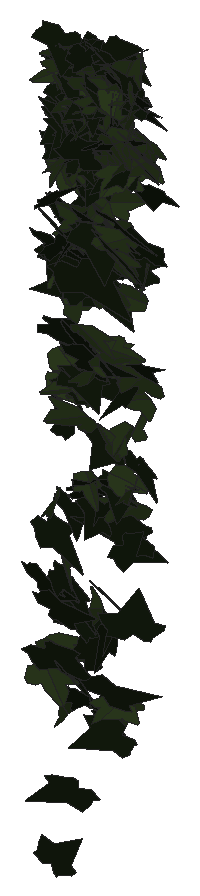
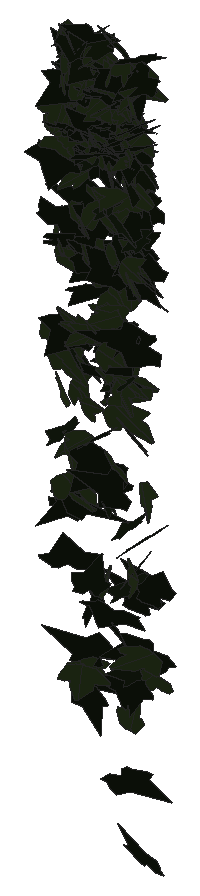
# SketchUp Ruby script. Lengths in millimetres.
U = 1.mm
M = Sketchup.active_model
def pt(a) = Geom::Point3d.new(a.map { |v| v * U })
def face(e, loops, mat)
  f = e.add_face(loops[0].map { |a| pt(a) })
  loops[1..].each { |l| e.add_face(l.map { |a| pt(a) }).erase! }
  f.material = f.back_material = mat if mat
  f
end
# faces: each face lists its corners as indices into pts; further lists are holes
def faces(e, pts, list, mat = nil) = list.each { |f| face(e, (f[0].is_a?(Array) ? f : [f]).map { |l| l.map { |i| pts[i] } }, mat) }
# xy, xz, yz: faces in a plane at the given z, y or x. An outline is a flat list of corners, or four numbers for a rectangle; further outlines are holes
def ring(l) = l.size == 4 ? [[l[0], l[1]], [l[2], l[1]], [l[2], l[3]], [l[0], l[3]]] : l.each_slice(2).to_a
def flat(e, list, mat, &to3) = list.each { |f| face(e, (f[0].is_a?(Array) ? f : [f]).map { |l| ring(l).map { |u, v| to3.(u, v) } }, mat) }
def xy(e, z, list, mat = nil) = flat(e, list, mat) { |x, y| [x, y, z] }
def xz(e, y, list, mat = nil) = flat(e, list, mat) { |x, z| [x, y, z] }
def yz(e, x, list, mat = nil) = flat(e, list, mat) { |y, z| [x, y, z] }
def lines(e, pts, list) = list.each { |a, b| e.add_line(pt(pts[a]), pt(pts[b])) }
# prism: a flat outline (further loops are holes) pulled along v
def prism(e, loops, v, mat = nil)
  f = face(e, loops, mat); d = Geom::Vector3d.new(v.map { |x| x * U })
  f.pushpull(f.normal.samedirection?(d) ? d.length : -d.length)
end
def box(e, o, s, mat = nil) = prism(e, [[o, [o[0] + s[0], o[1], o[2]], [o[0] + s[0], o[1] + s[1], o[2]], [o[0], o[1] + s[1], o[2]]]], [0, 0, s[2]], mat)
def at(x, y, z, deg = 0) = Geom::Transformation.translation(pt([x, y, z])) * Geom::Transformation.rotation(ORIGIN, Z_AXIS, deg.degrees)
def axes(o, x, y, z) = Geom::Transformation.new([*x, 0, *y, 0, *z, 0, *pt(o).to_a, 1])
def part(name) = M.definitions.add(name)
# library, detail: a bought-in or finely detailed component or shape, given as its bounding box
def library(name, o, s) = part(name).tap { |d| box(d.entities, o, s) }
def detail(e, o, s) = box(e.add_group.entities, o, s)
def put(e, d, t, mat = nil) = e.add_instance(d, t).tap { |i| i.material = mat if mat }
def group(e, t, mat = nil) = e.add_group.tap { |g| g.transformation = t; g.material = mat if mat }.entities
root = M.entities
M.materials.add("efeu1").color = [18, 25, 13]
M.materials.add("efeu2").color = [43, 57, 29]
c1 = part("ivyleaf_10")
p = [[0,12.8,-0.8],[-1.5,51.3,-10.9],[-4.9,51,-11.6],[-13.6,26.5,-7.3],[-13.2,15.9,-4.6],[-21.1,19.3,-7.2],
  [-29.5,16.3,-8.3],[-29.2,8.3,-6.2],[-19.7,-9.8,0.5],[-7.6,-13,4],[1,-12.2,5.8],[-0.4,51.1,-11.1],
  [-1.5,51.1,-10.9],[1,-12.4,5.9],[16.9,-12.4,3.5],[35.1,9.1,-5.1],[35,12.9,-6.1],[20.5,16.4,-4.9],
  [15.8,15,-3.8],[15.3,27.6,-7.1],[12.8,31.3,-7.8]]
faces(c1.entities,p,[[0,1,2,3,4,5,6,7,8,9,10],[11,12,0,13,14,15,16,17,18,19,20]],"efeu2")
c2 = part("ivyleaf_9")
p = [[39.1,54.8,31.7],[34.5,51.8,30.2],[-5.3,25.2,17.3],[-17.9,28.3,20.9],[-21.6,21.7,17],[-20.2,4.3,5.3],
  [-22.9,-0.3,2.5],[-17.1,-4,-0.6],[-2,-2.1,-1.2],[-0.7,-15.4,-10.1],[16.6,-22.3,-16.7],[21.1,-15.1,-12.5],
  [32.7,-10.7,-11],[46.1,-1.8,-6.6],[30.8,11.2,3.8]]
faces(c2.entities,p,[[0,1,2,3,4,5,6,7,8,9,10,11,12,13,14]],"efeu1")
put(root,c1,axes([2672.7,935.9,813.4],[0.15942,-0.86743,-0.26606],[-0.00895,0.26677,-0.87123],[1.72677,0.08147,0.02005]))
put(root,c2,axes([2720.5,938.2,1232.8],[-0.34672,-0.3779,-0.92751],[1.32636,0.62923,-0.39325],[1.36897,-0.70536,0.1461]))
put(root,c2,axes([2660.8,944.4,613.2],[0.17561,-0.06532,0.79458],[1.07748,-0.55783,-0.1116],[1.06836,0.57333,-0.01806]))
put(root,c2,axes([2787.7,950.3,434.8],[-1.28493,-0.29658,0.36083],[-0.63314,-0.13984,-0.7374],[0.62397,-0.75264,-0.00518]))
put(root,c1,axes([2677.2,946.4,1400.3],[0.03085,-0.75073,0.26481],[0.10097,-0.26326,-0.74957],[1.5117,0.0329,0.04466]))
put(root,c1,axes([2790.3,937.7,1478.8],[-1.40891,0.26566,-0.16374],[0.28464,-0.06793,-0.7864],[-0.52128,-0.75513,0.01314]))
put(root,c1,axes([2797,954.6,969.3],[-0.08285,-0.6242,0.55645],[0.28955,-0.55382,-0.60934],[1.56493,0.06942,0.1422]))
put(root,c1,axes([2822.4,927,1490],[0.29713,-0.25999,0.8628],[-0.7831,0.75847,0.303],[-1.52579,-0.43991,0.01251]))
put(root,c2,axes([2666.2,956.2,1276.6],[1.22665,-0.55319,-0.25391],[0.36613,-0.16572,0.84937],[-1.09906,-0.67262,-0.00044]))
put(root,c2,axes([2673.5,937.4,685.2],[0.65802,-0.47064,-0.52274],[-0.59753,0.41797,-0.58398],[1.19795,0.467,-0.00415]))
put(root,c2,axes([2657,928.9,1336.1],[0.09252,0.6858,-0.38367],[-0.11219,0.3865,0.6834],[1.49137,-0.01347,0.07521]))
put(root,c2,axes([2628.6,954.2,644.9],[0.27741,-0.22383,0.84752],[0.86326,-0.71593,-0.26709],[1.42759,0.47642,-0.00318]))
put(root,c1,axes([2702.9,956.9,1013.9],[-0.17582,-0.23371,0.79373],[-0.68279,-0.70837,-0.25033],[1.41902,-0.3698,-0.02211]))
put(root,c2,axes([2714.2,947.5,1067.5],[0.49529,-0.17699,0.81736],[1.30688,-0.44341,-0.31464],[0.90854,0.7343,0.00701]))
put(root,c1,axes([2725,942.1,1487.2],[0.18277,-0.80694,-0.22992],[-0.07025,0.22713,-0.81258],[1.59534,0.10245,-0.00944]))
put(root,c1,axes([2733.9,946.2,1050.5],[-0.37143,-0.74584,0.00108],[0.00403,-0.00167,-0.77095],[1.41948,-0.19516,0.00247]))
put(root,c2,axes([2716,947.6,1045.3],[-0.36467,-0.63332,-0.39148],[0.2294,0.37252,-0.66164],[1.39834,-0.22628,0.00645]))
put(root,c2,axes([2740.4,936.6,1617.8],[-0.89527,0.69738,0.26632],[-0.25461,0.23093,-0.84102],[-1.39773,-0.48875,-0.01738]))
put(root,c2,axes([2823.1,941,632.2],[-1.18983,-0.33633,0.57308],[1.1117,0.09693,0.69411],[-0.60287,0.84253,0.14891]))
put(root,c1,axes([2783.9,955.2,1533.3],[-0.17063,-0.77778,0.38312],[0.07826,-0.38854,-0.77916],[1.64824,-0.06207,0.07666]))
put(root,c1,axes([2826.6,929.7,1566.8],[0.06729,-0.15347,-0.87719],[-0.05514,0.87721,-0.15465],[1.69392,0.03465,0.02981]))
put(root,c2,axes([2787.1,958.1,1561.1],[-0.0691,-0.36872,0.77727],[0.87035,-0.66722,-0.29515],[1.38682,0.40036,0.22396]))
put(root,c2,axes([2709.5,947.5,1195.5],[-1.3001,0.31373,0.19461],[-0.34843,0.06757,-0.75157],[-0.61016,-0.70707,0.01452]))
put(root,c2,axes([2714.3,957.1,1463.5],[-1.48201,-0.3229,0.02286],[-0.03599,-0.01406,-0.84297],[0.61503,-0.7789,0.00574]))
put(root,c2,axes([2722.7,937.8,1429.1],[-0.27769,-0.00995,0.93928],[1.75685,0.17443,0.14524],[-0.33092,0.93441,-0.01711]))
put(root,c1,axes([2680.4,955.1,1564.4],[0.7392,0.38225,-0.66317],[-1.11093,-0.33316,-0.5339],[-0.9424,0.69257,0.10919]))
put(root,c2,axes([2731.9,945,1104],[1.36557,-0.37346,-0.34054],[-0.57379,0.15835,-0.80889],[0.77202,0.77828,0.00117]))
put(root,c2,axes([2723.4,949,548],[-0.37124,0.65819,0.57866],[0.2768,-0.56029,0.68632],[1.64482,0.24284,0.01511]))
put(root,c1,axes([2731.1,947.6,1560.2],[-1.35513,-0.2036,-0.34563],[0.65126,0.05915,-0.73979],[0.39837,-0.78927,0.03372]))
put(root,c1,axes([2696,958.5,1390.3],[0.17184,-0.75813,-0.35778],[0.37363,-0.33072,0.75033],[-1.55111,-0.16365,0.14111]))
put(root,c1,axes([2742.7,958.3,1526.1],[-0.52643,-0.71406,0.32298],[-0.07957,-0.32857,-0.76224],[1.48944,-0.26993,0.07343]))
put(root,c2,axes([2758.1,961.4,1279.5],[0.70383,-0.73572,0.38608],[0.39609,-0.3271,-0.82267],[1.53089,0.42288,0.03535]))
put(root,c1,axes([2722.5,950.5,1120.3],[-1.17375,0.19329,-0.48174],[0.88305,-0.13013,-0.6462],[-0.44291,-0.77168,-0.01169]))
put(root,c1,axes([2789.3,944.2,935.7],[0.68756,-0.16034,0.68765],[-1.21035,0.26174,0.39514],[-0.58391,-0.73134,-0.00934]))
put(root,c1,axes([2803.2,956.3,1482.5],[-1.05761,-0.327,0.56889],[-0.87459,-0.33821,-0.64328],[0.89145,-0.71976,0.04381]))
put(root,c1,axes([2715.5,958.8,854.4],[1.05753,-0.26871,0.55155],[0.93717,-0.24855,-0.61718],[0.69652,0.74241,-0.007]))
put(root,c2,axes([2739.4,963.1,1287.4],[-0.41817,-0.92359,-0.06457],[0.03619,0.06185,-0.94935],[1.76169,-0.2205,0.00417]))
put(root,c2,axes([2669.8,962.9,1615.3],[-0.58633,-0.77862,-0.02139],[0.02606,0.01758,-0.83733],[1.48221,-0.30831,0.00626]))
put(root,c2,axes([2789.6,939.3,1476.3],[0.837,0.67539,0.11118],[0.10284,0.09748,-0.80591],[-1.29863,0.44302,0.00783]))
put(root,c1,axes([2643.7,953.7,491.3],[1.49892,0.11324,0.37942],[0.71659,0.04721,-0.79566],[-0.23321,0.87293,-0.00619]))
put(root,c2,axes([2736.5,962.9,1559.2],[0.36434,-0.80566,0.1529],[0.03311,-0.15299,-0.8279],[1.56036,0.19137,-0.01814]))
put(root,c1,axes([2681.9,946.8,1066.9],[0.77895,0.63903,0.34305],[0.35015,0.28954,-0.75886],[-1.33521,0.44873,0.00112]))
put(root,c2,axes([2752.8,969.4,596.9],[-0.02818,0.03185,-0.97254],[1.18631,-0.74658,-0.03394],[-1.42207,-0.62344,-0.00904]))
put(root,c2,axes([2704.8,946,1111.4],[1.33807,-0.07472,-0.51763],[-0.9718,0.08956,-0.70646],[0.21534,0.86846,0.02832]))
put(root,c2,axes([2807.2,957,1047.6],[-1.17691,0.56372,-0.46815],[0.65936,-0.31487,-0.83677],[-1.22888,-0.70882,-0.00062]))
put(root,c2,axes([2648.2,948.7,534.5],[-0.1224,-0.04493,-0.85682],[1.17092,0.59647,-0.07746],[1.13818,-0.61846,-0.01246]))
put(root,c1,axes([2782.4,960.8,1298.4],[-0.85556,-0.26961,0.57998],[-0.77328,-0.42711,-0.51347],[0.94009,-0.59669,0.10548]))
put(root,c2,axes([2783.6,958.5,1422.2],[-1.27403,0.28651,-0.3096],[0.49768,-0.17384,-0.72627],[-0.62996,-0.71677,0.05238]))
put(root,c1,axes([2782.5,958.8,1413],[1.0057,0.51896,-0.39533],[-0.58093,-0.25295,-0.74005],[-1.09733,0.60954,0.02947]))
put(root,c1,axes([2758.8,950.7,1209.2],[-1.70865,0.06043,0.2919],[-0.5547,0.01631,-0.8998],[-0.11897,-0.9439,0.00314]))
put(root,c2,axes([2759.5,961.1,1320],[0.78526,-0.46789,0.54841],[0.77524,-0.37002,-0.62216],[1.13198,0.57799,0.04565]))
put(root,c1,axes([2692.4,949.4,1557.1],[-0.80403,-0.11546,-0.7096],[1.32313,0.14407,-0.43734],[0.34858,-0.81318,0.02327]))
put(root,c1,axes([2718,953.3,1499.1],[-0.54373,-0.77837,-0.12874],[0.08638,0.12048,-0.82914],[1.49903,-0.28927,0.00108]))
put(root,c1,axes([2703.8,968.5,1305.9],[-0.72792,-0.4744,-0.72554],[-0.85098,-0.57142,0.60934],[-1.41341,0.58836,0.00679]))
put(root,c1,axes([2739.5,953.7,1448.3],[-1.22505,0.46513,-0.12795],[0.18629,-0.08298,-0.79409],[-0.89901,-0.65101,0.00981]))
put(root,c1,axes([2801.2,956.6,1612.9],[-0.82733,-0.70588,0.01715],[-0.01854,-0.01415,-0.82899],[1.3437,-0.43481,-0.00087]))
put(root,c1,axes([2760.1,946.1,1072.6],[-0.2766,-0.34891,0.74435],[0.70572,0.6468,0.37558],[-1.39634,0.39601,0.04237]))
put(root,c2,axes([2752,954.2,491.6],[0.18914,-0.0196,0.83537],[1.53631,-0.21511,-0.10108],[0.4109,0.81329,-0.00661]))
put(root,c1,axes([2783.2,942.1,1536.1],[0.44676,0.64527,-0.63514],[0.1941,0.63312,0.68091],[1.71223,-0.24014,0.08853]))
put(root,c1,axes([2827.3,956.7,1448.2],[-1.23998,0.00173,0.47916],[-0.9028,-0.11656,-0.64458],[0.1288,-0.80031,0.09491]))
put(root,c2,axes([2727.8,973.7,791.9],[-0.30813,-0.59527,0.53616],[-0.27348,-0.51655,-0.61689],[1.49999,-0.21646,-0.00234]))
put(root,c1,axes([2812.8,958.7,1203.8],[-0.16965,0.00393,-0.79023],[-1.50347,0.02042,0.08921],[0.03946,0.79498,0.00162]))
put(root,c2,axes([2689.4,966.3,299.2],[0.04421,0.06156,-0.80436],[-0.5756,-0.74534,-0.06577],[-1.42336,0.30332,0.00162]))
put(root,c2,axes([2644.2,958.3,749.8],[0.58112,-0.83208,-0.39431],[-0.20035,0.38115,-0.88583],[1.74093,0.32161,0.02968]))
put(root,c1,axes([2730.3,969.9,628.5],[-0.39409,0.37062,0.7211],[0.58023,-0.65404,0.4237],[1.42981,0.36757,0.02681]))
put(root,c2,axes([2725.3,966,1575.4],[-0.66683,-0.70614,-0.2528],[0.45866,0.15824,-0.77601],[1.35177,-0.40203,0.1386]))
put(root,c2,axes([2680.1,944,1428.1],[-0.29968,0.63778,0.51889],[-0.32559,0.49135,-0.65583],[-1.53056,-0.2294,0.03792]))
put(root,c2,axes([2804.3,968,1582.8],[-0.01937,-0.94154,0.03423],[0.01272,0.03416,0.94158],[-1.79308,0.01042,0.00631]))
put(root,c1,axes([2823.3,956.8,1068.5],[-1.62784,-0.0793,0.43208],[-0.81798,-0.04455,-0.85897],[0.17293,-0.95722,0.00418]))
put(root,c2,axes([2710.8,970.8,1521.2],[-0.10955,-0.81263,0.14807],[-0.05328,-0.14642,-0.81448],[1.57115,-0.06163,-0.0173]))
put(root,c1,axes([2772.4,964.6,474.6],[1.0681,0.4258,-0.46867],[-0.71452,-0.28056,-0.70446],[-0.97047,0.67521,0.00284]))
put(root,c1,axes([2771.3,958.1,1266.6],[-1.32442,0.12671,-0.34042],[0.61959,-0.10874,-0.70597],[-0.30663,-0.76702,0.04385]))
put(root,c2,axes([2671.3,968.8,652.7],[0.57538,-0.90792,0.12651],[0.08216,-0.11897,-0.95693],[1.74271,0.30537,0.00335]))
put(root,c2,axes([2774.8,949.6,1512.1],[0.07015,-0.37409,0.75682],[0.49263,0.72606,0.34628],[-1.52934,0.21672,0.14626]))
put(root,c2,axes([2700.2,976.1,1490.8],[-0.58174,-0.62853,0.46493],[0.15563,-0.52217,-0.65214],[1.47975,-0.19218,0.25137]))
put(root,c1,axes([2716.3,943.6,1020.7],[0.34793,0.24503,-0.78762],[0.64119,0.7142,0.30038],[1.43296,-0.37907,0.05683]))
put(root,c2,axes([2739.1,973.2,1523.8],[-1.28127,-0.40069,0.27581],[-0.30363,-0.26301,-0.77151],[0.87459,-0.67832,0.13622]))
put(root,c2,axes([2659.2,967.5,1313],[1.2524,-0.06727,-0.51152],[0.96347,-0.07573,0.66121],[-0.1894,-0.83003,-0.01888]))
put(root,c2,axes([2695.7,968.9,1286.3],[-0.64733,0.42247,-0.77528],[0.90343,-0.61303,-0.54231],[-1.41684,-0.58391,0.00842]))
put(root,c1,axes([2809.9,961.5,1530.4],[0.05668,-0.835,-0.01775],[-0.01542,0.01748,-0.83549],[1.58945,0.02995,-0.00747]))
put(root,c2,axes([2688.5,959.3,1549.6],[0.61306,-0.68183,-0.35126],[-0.14218,0.35128,-0.75038],[1.4528,0.3221,0.07479]))
put(root,c1,axes([2815.1,963.1,1617.3],[0.17058,-0.82463,0.07011],[0.44247,-0.04259,-0.79818],[1.51167,0.10552,0.22572]))
put(root,c2,axes([2802,966.3,1552.2],[-1.56301,-0.03334,-0.01598],[0.03086,-0.0054,-0.82191],[0.06324,-0.82139,0.00605]))
put(root,c1,axes([2786.7,962.7,1430.3],[-1.2637,-0.63073,0.06055],[0.09244,0.03678,0.91578],[-1.20237,0.66573,0.00677]))
put(root,c1,axes([2699.8,961.6,957.9],[-1.07253,-0.19468,0.67021],[-1.22089,-0.1948,-0.59598],[0.52317,-0.85371,-0.01684]))
put(root,c2,axes([2696.6,975.5,1015.9],[0.79633,-0.76132,-0.18772],[0.19844,-0.15686,0.86858],[-1.47908,-0.43094,0.01546]))
put(root,c1,axes([2680.7,959.4,1595.5],[-1.01355,-0.62878,-0.11069],[0.10024,0.10039,-0.82363],[1.21095,-0.53459,-0.02447]))
put(root,c2,axes([2780.8,969,1461.5],[0.7426,-0.6508,0.27175],[0.33325,-0.21145,-0.7578],[1.30023,0.42589,0.03902]))
put(root,c1,axes([2803.6,955.2,1446.8],[-0.22263,-0.72728,-0.411],[0.09085,0.40851,-0.73646],[1.58729,-0.12539,-0.01549]))
put(root,c2,axes([2678.3,948.2,1400],[0.32565,0.75323,0.1979],[0.0868,0.19258,-0.77241],[-1.47965,0.17707,-0.00175]))
put(root,c1,axes([2665.3,960.7,1474.7],[-1.40582,0.29447,-0.24979],[0.42623,-0.11254,-0.79493],[-0.59869,-0.77159,0.02061]))
put(root,c2,axes([2667.4,946.3,1258.2],[-0.12875,0.11804,-0.82061],[-0.49208,0.77927,0.13341],[1.49916,0.26592,-0.02669]))
put(root,c1,axes([2755.1,962.2,1580.5],[-1.11668,-0.60124,-0.00818],[0.00861,0.00701,-0.84008],[1.14434,-0.58675,-0.00166]))
put(root,c2,axes([2758.5,959.5,1630.4],[-0.19763,-0.39536,-0.73817],[0.73401,0.63766,-0.39578],[1.4146,-0.3861,0.10223]))
put(root,c1,axes([2676.2,963.2,1187.8],[1.00666,0.56042,-0.0564],[-0.07579,-0.03997,-0.77061],[-1.06931,0.53043,0.00153]))
put(root,c2,axes([2797.1,969.2,1557],[-1.54014,-0.03063,0.18632],[-0.35454,-0.00429,-0.80981],[0.05864,-0.8304,-0.00269]))
put(root,c2,axes([2739.3,968.7,1393.9],[-1.30451,0.07223,-0.39946],[0.76189,-0.00967,-0.68866],[-0.12807,-0.79327,-0.02798]))
put(root,c1,axes([2803.2,960.2,866.6],[-0.02823,-0.78479,-0.29344],[-0.0224,0.29365,-0.78476],[1.59445,-0.00977,-0.01622]))
put(root,c2,axes([2762.7,960.9,1459.1],[0.12892,0.75149,-0.39845],[-0.05733,-0.39734,-0.75452],[-1.61782,0.07396,-0.00501]))
put(root,c2,axes([2663.2,969.7,1227],[-1.30621,0.01807,-0.40688],[0.77397,-0.01322,-0.68656],[-0.04242,-0.79775,0.00216]))
put(root,c2,axes([2714,955.6,1443.5],[0.93502,0.07557,-0.68058],[-1.30288,0.07407,-0.48594],[0.03091,0.8361,0.10457]))
put(root,c1,axes([2750.6,963.5,1597.2],[-0.47535,-0.79687,-0.10201],[0.01983,0.1036,-0.83484],[1.52886,-0.24911,-0.02089]))
put(root,c2,axes([2647.1,963,156],[-0.61439,0.52243,0.57369],[0.57643,-0.48723,0.61412],[1.35958,0.44266,-0.00112]))
put(root,c2,axes([2763.7,969.4,1477.8],[1.02723,-0.51827,0.31041],[0.44085,-0.2069,-0.74821],[1.06189,0.58725,0.01034]))
put(root,c1,axes([2694.7,947.6,1163.1],[0.18867,-0.15937,-0.9898],[0.86749,0.89306,-0.09814],[1.69946,-0.43817,0.15998]))
put(root,c2,axes([2702.2,973.9,1451.2],[-0.55447,-0.85831,-0.02374],[0.04662,-0.03337,0.90577],[-1.63349,0.29039,0.03391]))
put(root,c1,axes([2686.5,959.9,1508.5],[-0.57547,-0.66513,-0.40057],[0.33685,0.35951,-0.73055],[1.43881,-0.35019,0.01082]))
put(root,c2,axes([2629.2,972.3,1230.7],[0.6293,-0.32867,0.68533],[1.00468,-0.43841,-0.46494],[1.04076,0.62194,0.03443]))
put(root,c1,axes([2782.5,969,1557.9],[-0.55365,-0.77456,0.09112],[-0.06542,-0.08443,-0.82738],[1.48286,-0.29292,-0.00248]))
put(root,c2,axes([2718.9,970.2,1410.2],[-0.35618,-0.69432,-0.37775],[0.2938,0.34862,-0.71724],[1.47538,-0.23704,0.05163]))
put(root,c2,axes([2675,981.6,1454.9],[-0.92796,-0.49086,0.40875],[-0.39711,-0.36362,-0.68556],[1.149,-0.5221,0.09317]))
put(root,c1,axes([2741.8,967,1342.3],[1.30622,-0.48896,-0.21172],[-0.31459,0.13283,-0.84261],[0.96405,0.70585,0.0119]))
put(root,c2,axes([2753,957.7,1449.7],[1.33199,0.37017,-0.14344],[-0.24577,-0.06263,-0.79172],[-0.71446,0.71166,0.00493]))
put(root,c2,axes([2680.5,960.7,473],[1.18624,0.16239,-0.47769],[-0.88953,-0.10012,-0.64388],[-0.36166,0.77888,0.01683]))
put(root,c1,axes([2758.2,973.9,1089.4],[0.35048,-0.12462,-0.79228],[1.25221,-0.44138,0.22236],[-0.87287,-0.68323,0.00087]))
put(root,c2,axes([2733.4,962.2,1011.7],[-1.77496,-0.15857,0.03687],[0.07405,-0.00889,0.94588],[-0.30086,0.93331,0.01528]))
put(root,c1,axes([2779.6,968.9,1528.8],[-1.3024,-0.35081,0.31177],[-0.53532,-0.13471,-0.76896],[0.71504,-0.73983,-0.00782]))
put(root,c2,axes([2729.4,966.7,1294.9],[-0.27717,-0.48482,-0.63158],[0.61819,0.55002,-0.49712],[1.3835,-0.3429,0.0956]))
put(root,c1,axes([2741.1,968.3,1545.8],[1.25098,0.51168,-0.01222],[-0.00432,-0.01698,-0.8329],[-0.97409,0.6572,-0.012]))
put(root,c2,axes([2760.4,981.8,847.3],[-0.19257,-0.76423,0.26964],[-0.08564,-0.26602,-0.77085],[1.53999,-0.11036,-0.00915]))
put(root,c2,axes([2738,969.9,1599.6],[0.64863,-0.74131,-0.22969],[0.00506,0.25197,-0.80929],[1.47703,0.32468,0.10364]))
put(root,c2,axes([2653,973.8,508.5],[0.86972,-0.68723,0.10637],[0.10679,-0.09042,-0.82529],[1.3192,0.4604,-0.00332]))
put(root,c1,axes([2793.3,969.3,1573.9],[-0.45058,-0.80375,-0.01503],[-0.03545,0.02115,-0.83755],[1.52955,-0.23628,-0.02384]))
put(root,c2,axes([2728.9,965.4,1620],[1.24871,-0.52744,-0.15759],[0.07101,0.28724,-0.80599],[1.04526,0.61058,0.24303]))
put(root,c1,axes([2809.2,970.1,1613.8],[0.90659,-0.69796,-0.05806],[0.09133,0.10258,-0.83941],[1.32981,0.46879,0.09723]))
put(root,c2,axes([2732.3,957.3,853.6],[1.48467,0.50436,0.10851],[0.17163,0.06037,-0.92893],[-0.96675,0.78528,0.00172]))
put(root,c1,axes([2727.3,967.2,1578.5],[-0.93086,0.66794,-0.01702],[0.03044,-0.00938,-0.82784],[-1.27127,-0.48931,-0.00736]))
put(root,c2,axes([2778.2,975.9,1412.9],[-1.5218,0.04977,-0.03695],[0.06969,-0.00639,-0.80114],[-0.09517,-0.80043,0.0041]))
put(root,c2,axes([2684.9,980.6,1495.7],[-0.99563,-0.61164,-0.14091],[0.29102,0.05372,-0.80085],[1.15858,-0.53911,0.08007]))
put(root,c1,axes([2656.4,983.2,680.9],[-0.33101,0.41093,-0.79478],[0.42821,-0.76355,-0.44402],[-1.64813,-0.28091,0.04426]))
put(root,c1,axes([2639.2,978,1375],[0.61695,-0.23855,-0.75403],[1.14567,-0.4541,0.40246],[-0.9762,-0.68369,-0.00421]))
put(root,c1,axes([2763.6,971.7,1549.9],[-0.38321,0.7831,-0.18149],[-0.07739,-0.19678,-0.80396],[-1.52794,-0.18644,0.08624]))
put(root,c1,axes([2697.8,971.7,1510.8],[0.98245,0.64006,-0.07904],[-0.0784,-0.0683,-0.82221],[-1.22491,0.51774,-0.01076]))
put(root,c2,axes([2649.4,963.1,1098.5],[0.63094,0.35086,-0.79637],[1.08639,0.55558,0.48239],[1.25014,-0.65988,-0.01728]))
put(root,c2,axes([2651.9,977.6,1560.9],[0.31924,-0.80844,-0.10977],[0.0285,0.1151,-0.8248],[1.55249,0.16413,0.03771]))
put(root,c1,axes([2703.2,965.3,1545.6],[-1.04667,0.32991,0.52388],[-0.95751,0.17023,-0.63534],[-0.68669,-0.74022,0.08739]))
put(root,c2,axes([2681.6,961.9,1450.1],[0.52274,0.74943,-0.05917],[-0.01182,-0.06074,-0.79804],[-1.43071,0.27433,-0.01503]))
put(root,c1,axes([2709.4,968.3,1024.8],[0.54533,-0.07436,-0.73317],[-1.28143,0.29334,-0.29289],[0.5701,0.73047,0.04298]))
put(root,c2,axes([2791.1,975.8,1615.9],[-0.69681,0.57412,-0.48783],[0.10187,-0.52119,-0.65356],[-1.43023,-0.31684,0.19112]))
put(root,c2,axes([2795,959.7,1076.8],[1.13092,0.51481,0.15954],[0.23544,0.10085,-0.7862],[-0.99838,0.60694,-0.00468]))
put(root,c1,axes([2661.1,985,414.8],[-0.32739,-0.60054,-0.57502],[-0.17545,-0.5698,0.62267],[-1.57265,0.18859,0.05024]))
put(root,c2,axes([2748.9,977.3,1231],[-0.08426,0.46053,-0.64789],[-0.09186,-0.64925,-0.4582],[-1.51004,0.0138,0.06402]))
put(root,c2,axes([2644.1,966.9,1593.6],[1.48631,-0.19101,-0.22358],[-0.3946,0.09226,-0.80303],[0.39687,0.80707,0.03888]))
put(root,c1,axes([2780.5,958.1,880.7],[0.15598,0.53616,0.69382],[0.23527,0.68282,-0.54226],[-1.65214,0.14785,-0.01172]))
put(root,c2,axes([2686.1,968.6,1576.6],[0.77528,0.52376,-0.51659],[-0.63783,-0.39355,-0.66328],[-1.24638,0.52719,0.0181]))
put(root,c1,axes([2814.9,979.2,1246.4],[0.68365,-0.63716,0.27491],[0.35735,-0.20877,-0.72921],[1.27143,0.40128,0.05713]))
put(root,c1,axes([2808.8,973,1481],[-0.95594,0.58687,-0.24284],[0.2629,-0.20124,-0.77207],[-1.17983,-0.52034,0.02472]))
put(root,c1,axes([2759.5,975.9,1537.4],[-0.94632,-0.63579,0.18275],[-0.16876,-0.16249,-0.8066],[1.24767,-0.50421,0.02951]))
put(root,c1,axes([2714.3,985,1071.5],[-0.13417,-0.58034,0.57005],[-0.04003,-0.57069,-0.5836],[1.5477,-0.06507,0.03433]))
put(root,c1,axes([2665.2,974.1,1549.4],[0.17162,-0.83085,-0.06296],[-0.01171,0.06266,-0.83573],[1.58576,0.09038,0.00064]))
put(root,c1,axes([2783.3,955.2,1364.8],[0.07148,0.22478,0.87782],[-0.09189,0.87782,-0.22272],[-1.72212,-0.03751,0.04832]))
put(root,c1,axes([2760.5,984.5,1445.3],[-0.49383,0.12107,-0.74777],[0.66476,-0.68226,-0.23167],[-1.27929,-0.40126,0.16827]))
put(root,c2,axes([2730.2,981.2,1421.2],[-1.4562,-0.20804,-0.00468],[0.00893,0.0006,-0.79291],[0.39594,-0.76514,0.00065]))
put(root,c1,axes([2747.5,979,1298.9],[-1.50456,-0.25636,-0.33552],[-0.58368,-0.1409,0.83027],[-0.55238,0.84716,0.03656]))
put(root,c1,axes([2676.9,963.4,992.6],[1.07774,0.63153,-0.45624],[0.58811,0.3357,0.84822],[1.36115,-0.64508,-0.00524]))
put(root,c2,axes([2660.8,986.6,1500.3],[-0.25587,-0.77943,0.18187],[-0.06722,-0.17846,-0.79093],[1.52177,-0.13894,-0.00436]))
put(root,c2,axes([2739.9,983.6,1536.8],[-1.45034,-0.29351,-0.10316],[0.23065,-0.02869,-0.81364],[0.54534,-0.76847,0.06977]))
put(root,c1,axes([2737.8,980.2,1432.6],[0.92222,-0.49437,0.40007],[0.77912,-0.14245,-0.67185],[0.92629,0.61202,0.16679]))
put(root,c1,axes([2658,975.3,1234.5],[-0.78612,-0.03071,-0.64357],[1.20506,-0.16078,-0.39871],[-0.22685,-0.74762,0.11218]))
put(root,c1,axes([2708.1,964.5,1473.8],[0.57227,-0.32883,-0.7679],[-0.75572,0.66177,-0.43886],[1.39872,0.49209,0.07706]))
put(root,c1,axes([2699.1,969.2,1011.2],[0.99612,-0.43675,-0.50405],[-0.52098,0.44359,-0.66861],[1.15748,0.57552,0.13283]))
put(root,c2,axes([2792.1,960.3,764.7],[0.28274,-0.10795,-0.88524],[-0.38981,0.86931,-0.14039],[1.65189,0.22362,0.11839]))
put(root,c2,axes([2730,983.4,1451.5],[-1.31007,-0.06817,-0.44222],[0.85136,-0.08676,-0.68294],[0.01898,-0.81355,0.10989]))
put(root,c2,axes([2739.9,959.2,799.4],[-0.07871,0.52449,0.64819],[-0.08053,0.64683,-0.52609],[-1.58487,-0.05891,-0.00546]))
put(root,c2,axes([2815.5,985.4,1244.2],[-0.93462,-0.03856,0.61642],[-1.1024,-0.24455,-0.47676],[0.40794,-0.74921,0.12389]))
put(root,c1,axes([2814.2,970.9,1024.3],[1.02757,-0.15425,-0.6199],[-0.98295,0.37225,-0.54246],[0.71547,0.73295,0.14504]))
put(root,c2,axes([2701,980.8,605.1],[-0.96055,-0.43084,-0.58721],[0.95091,0.31499,-0.66054],[1.00852,-0.70734,0.06352]))
put(root,c2,axes([2735.9,993.2,908.2],[-0.50969,-0.6092,0.50502],[-0.34065,-0.47271,-0.66513],[1.46699,-0.32143,0.02101]))
put(root,c2,axes([2759.3,969.6,430.7],[0.77523,0.01432,-0.74102],[-1.41054,0.00184,-0.40736],[-0.01006,0.84559,0.01343]))
put(root,c2,axes([2736.2,961.8,1225.8],[0.9915,0.52981,0.32483],[0.40695,0.24517,-0.74282],[-1.11054,0.56286,0.01781]))
put(root,c1,axes([2740.4,979.3,1455.9],[1.41495,-0.33584,-0.01719],[-0.02835,0.00878,-0.81579],[0.63938,0.74361,0.00187]))
put(root,c2,axes([2639.1,976.2,1305.2],[0.98114,-0.56819,-0.21912],[-0.23691,0.18271,-0.76664],[1.13453,0.52952,0.02941]))
put(root,c1,axes([2692.2,985.6,1270.1],[-0.23297,-0.65733,0.39168],[-0.11067,-0.38752,-0.66853],[1.45208,-0.135,0.01189]))
put(root,c2,axes([2733.2,987.7,1281.2],[0.29734,-0.34816,0.71213],[0.71267,-0.60732,-0.37907],[1.32968,0.40336,0.04393]))
put(root,c1,axes([2747,967.9,1089.2],[0.6595,0.45787,0.5904],[0.65529,0.47972,-0.57412],[-1.26196,0.48838,0.01042]))
put(root,c2,axes([2802,982.3,773.8],[-0.74483,-0.27666,-0.767],[-1.19008,-0.44417,0.47927],[-0.99591,0.73768,0.00092]))
put(root,c1,axes([2744.1,984.3,1432],[-0.6385,0.45021,-0.56808],[0.55159,-0.49044,-0.55984],[-1.26446,-0.44128,0.04264]))
put(root,c2,axes([2721,970.7,991],[-0.11163,-0.44691,0.68422],[0.24484,0.67238,0.4502],[-1.53598,0.13966,0.02204]))
put(root,c2,axes([2793.5,988.2,899.9],[0.34996,-0.75119,0.21431],[0.09326,-0.20864,-0.77337],[1.48378,0.19029,-0.00194]))
put(root,c2,axes([2804.1,986.3,1455.7],[-1.47431,-0.11588,0.15157],[-0.26368,-0.09409,-0.78002],[0.24965,-0.78371,0.07124]))
put(root,c1,axes([2800.5,978.5,960.5],[0.78182,-0.71874,-0.00644],[0.00787,-0.00506,0.82785],[-1.36794,-0.41081,0.00108]))
put(root,c2,axes([2736.1,969,1455.2],[-0.55268,-0.13822,0.83068],[1.51705,0.23827,0.3183],[-0.51689,0.84711,0.04601]))
put(root,c1,axes([2817.1,974.1,1477.1],[-1.40862,0.35899,0.06304],[-0.10324,0.03261,-0.82258],[-0.68595,-0.74209,-0.00565]))
put(root,c1,axes([2789.7,969.5,1255.6],[-0.76607,0.28022,0.67404],[-1.15168,0.3024,-0.48708],[-0.77699,-0.7245,0.0574]))
put(root,c2,axes([2688.1,975.4,1223.3],[1.29364,0.43854,-0.38088],[0.59234,0.22004,0.80878],[0.93339,-0.74744,0.01463]))
put(root,c2,axes([2740.6,989.3,636],[1.05178,-0.55946,0.01026],[-0.01373,0.00729,0.78638],[-1.06485,-0.55268,-0.00001]))
put(root,c1,axes([2671.4,979.2,1439.9],[0.17274,0.79865,-0.1311],[-0.33339,-0.10941,-0.78779],[-1.50382,0.11599,0.15959]))
put(root,c2,axes([2728.7,985.8,1424.7],[0.72832,-0.68496,0.13393],[0.16767,-0.10412,-0.78419],[1.31767,0.39185,0.02575]))
put(root,c1,axes([2642.2,972.6,537.3],[-0.92674,-0.30004,-0.64164],[1.11029,0.27173,-0.56979],[0.76459,-0.75827,0.0497]))
put(root,c2,axes([2697.5,987.7,1345.1],[0.50067,-0.72725,0.15455],[0.14805,-0.13612,-0.77292],[1.40725,0.27306,0.02633]))
put(root,c2,axes([2651.6,984.1,1221.6],[-0.97688,-0.13106,-0.61206],[1.12671,0.15542,-0.52975],[0.38689,-0.78353,-0.0027]))
put(root,c1,axes([2702.6,985.7,1408.7],[0.46354,-0.71246,0.24762],[0.38799,-0.18835,-0.74243],[1.38209,0.29183,0.12537]))
put(root,c1,axes([2763.6,981.9,1294.3],[0.64026,-0.73358,-0.02461],[-0.01794,0.02275,-0.80704],[1.39682,0.33654,0.00092]))
put(root,c2,axes([2682.1,967.8,935.3],[-0.96366,0.20726,-0.59662],[-1.04952,0.22772,0.54712],[0.58603,0.74865,-0.00125]))
put(root,c1,axes([2657.7,969.2,1559.5],[0.15086,0.67426,0.48615],[0.11855,0.48217,-0.67889],[-1.57758,0.10071,-0.00453]))
put(root,c2,axes([2735.5,987.8,1436.7],[-1.49211,-0.13139,0.02958],[-0.05903,0.00614,-0.79486],[0.24944,-0.78454,-0.01117]))
put(root,c2,axes([2734.2,993.4,1430.4],[-0.89645,-0.64152,0.0691],[0.09131,-0.12014,-0.78832],[1.22461,-0.46066,0.10937]))
put(root,c2,axes([2781.6,972.6,1532.7],[1.57432,0.06653,-0.0089],[-0.02803,0.07252,-0.82661],[-0.12464,0.82406,0.07346]))
put(root,c1,axes([2804.5,983.3,1426.3],[1.2677,0.24438,-0.3358],[-0.65706,-0.02695,-0.70444],[-0.43934,0.74546,0.08461]))
put(root,c2,axes([2657.4,996.2,773.8],[0.0218,-0.7154,0.3866],[0.00046,-0.38663,-0.71547],[1.54763,0.01019,-0.00523]))
put(root,c2,axes([2756.4,965,1583.7],[0.68711,0.60133,0.45345],[0.35043,0.41712,-0.69976],[-1.38988,0.40245,0.04774]))
put(root,c2,axes([2816.7,975.8,1395.5],[1.26538,0.22568,-0.35782],[-0.63447,-0.13085,-0.70197],[-0.49568,0.74361,-0.01492]))
put(root,c1,axes([2765.2,980.1,468.4],[-1.17529,-0.59334,-0.12628],[0.17328,0.0875,-0.85639],[1.14147,-0.62421,-0.00002]))
put(root,c1,axes([2661.7,992.1,1250.9],[-0.1771,-0.60945,0.4536],[-0.02286,-0.45575,-0.6148],[1.44572,-0.08187,0.04584]))
put(root,c2,axes([2811.6,980.5,1273],[0.74699,-0.24506,0.67965],[-0.83711,0.53257,0.44603],[-1.09086,-0.5765,0.12313]))
put(root,c2,axes([2691.8,971.1,820.6],[0.63837,0.66325,-0.38538],[0.21162,0.37413,0.74067],[1.4445,-0.34792,0.06181]))
put(root,c1,axes([2737.4,980.8,1518],[-1.42986,0.20702,-0.27007],[0.49415,-0.07439,-0.77929],[-0.41863,-0.79489,0.00259]))
put(root,c1,axes([2659.2,987.5,1232],[0.40008,-0.77706,0.13069],[0.07641,-0.12452,-0.80497],[1.49773,0.21393,0.00616]))
put(root,c1,axes([2678.7,977.9,1364.2],[1.19551,0.40018,0.47026],[0.70178,0.29497,-0.74356],[-0.94264,0.72713,0.04283]))
put(root,c2,axes([2702.6,982,1326.9],[-1.03073,0.59167,-0.14623],[0.19008,-0.10683,-0.80211],[-1.14427,-0.55071,-0.00152]))
put(root,c1,axes([2781.9,990,815.5],[-1.01469,-0.60408,0.47024],[-0.59991,-0.34899,-0.80569],[1.32772,-0.61934,-0.00466]))
put(root,c1,axes([2700.4,990,1190.4],[0.24826,0.61784,-0.43367],[-0.41984,-0.38968,-0.62153],[-1.37391,0.23072,0.11156]))
put(root,c2,axes([2732.6,984.4,1184],[-0.17265,-0.65346,-0.51776],[0.2839,0.49969,-0.65679],[1.56114,-0.16314,0.06218]))
